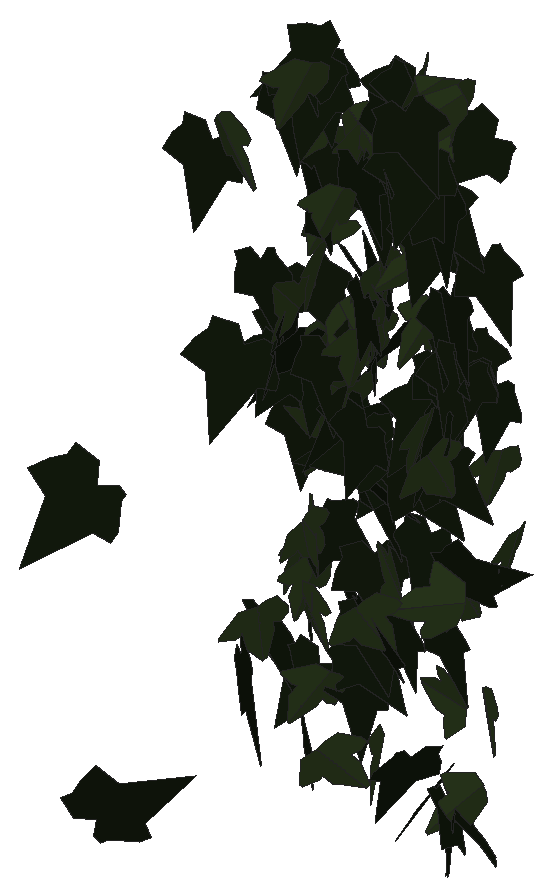
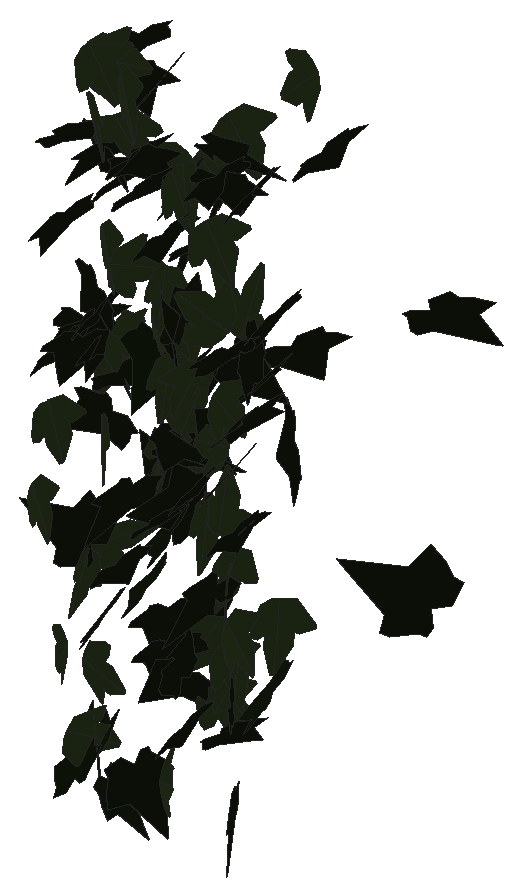
# SketchUp Ruby script. Lengths in inches.
U = 1.inch
M = Sketchup.active_model
def pt(a) = Geom::Point3d.new(a.map { |v| v * U })
def face(e, loops, mat)
  f = e.add_face(loops[0].map { |a| pt(a) })
  loops[1..].each { |l| e.add_face(l.map { |a| pt(a) }).erase! }
  f.material = f.back_material = mat if mat
  f
end
# faces: each face lists its corners as indices into pts; further lists are holes
def faces(e, pts, list, mat = nil) = list.each { |f| face(e, (f[0].is_a?(Array) ? f : [f]).map { |l| l.map { |i| pts[i] } }, mat) }
# xy, xz, yz: faces in a plane at the given z, y or x. An outline is a flat list of corners, or four numbers for a rectangle; further outlines are holes
def ring(l) = l.size == 4 ? [[l[0], l[1]], [l[2], l[1]], [l[2], l[3]], [l[0], l[3]]] : l.each_slice(2).to_a
def flat(e, list, mat, &to3) = list.each { |f| face(e, (f[0].is_a?(Array) ? f : [f]).map { |l| ring(l).map { |u, v| to3.(u, v) } }, mat) }
def xy(e, z, list, mat = nil) = flat(e, list, mat) { |x, y| [x, y, z] }
def xz(e, y, list, mat = nil) = flat(e, list, mat) { |x, z| [x, y, z] }
def yz(e, x, list, mat = nil) = flat(e, list, mat) { |y, z| [x, y, z] }
def lines(e, pts, list) = list.each { |a, b| e.add_line(pt(pts[a]), pt(pts[b])) }
# prism: a flat outline (further loops are holes) pulled along v
def prism(e, loops, v, mat = nil)
  f = face(e, loops, mat); d = Geom::Vector3d.new(v.map { |x| x * U })
  f.pushpull(f.normal.samedirection?(d) ? d.length : -d.length)
end
def box(e, o, s, mat = nil) = prism(e, [[o, [o[0] + s[0], o[1], o[2]], [o[0] + s[0], o[1] + s[1], o[2]], [o[0], o[1] + s[1], o[2]]]], [0, 0, s[2]], mat)
def at(x, y, z, deg = 0) = Geom::Transformation.translation(pt([x, y, z])) * Geom::Transformation.rotation(ORIGIN, Z_AXIS, deg.degrees)
def axes(o, x, y, z) = Geom::Transformation.new([*x, 0, *y, 0, *z, 0, *pt(o).to_a, 1])
def part(name) = M.definitions.add(name)
# library, detail: a bought-in or finely detailed component or shape, given as its bounding box
def library(name, o, s) = part(name).tap { |d| box(d.entities, o, s) }
def detail(e, o, s) = box(e.add_group.entities, o, s)
def put(e, d, t, mat = nil) = e.add_instance(d, t).tap { |i| i.material = mat if mat }
def group(e, t, mat = nil) = e.add_group.tap { |g| g.transformation = t; g.material = mat if mat }.entities
root = M.entities
M.materials.add("efeu1").color = [18, 25, 13]
M.materials.add("efeu2").color = [43, 57, 29]
c1 = part("ivyleaf_9")
p = [[1.54,2.16,1.25],[1.36,2.04,1.19],[-0.21,0.99,0.68],[-0.71,1.11,0.82],[-0.85,0.86,0.67],[-0.8,0.17,0.21],
  [-0.9,-0.01,0.1],[-0.67,-0.16,-0.02],[-0.08,-0.08,-0.05],[-0.03,-0.6,-0.4],[0.65,-0.88,-0.66],[0.83,-0.6,-0.49],
  [1.29,-0.42,-0.43],[1.8125,-0.07,-0.26],[1.21,0.44,0.15]]
faces(c1.entities,p,[[0,1,2,3,4,5,6,7,8,9,10,11,12,13,14]],"efeu1")
c2 = part("ivyleaf_10")
p = [[0,0.5,-0.03],[-0.0625,2.02,-0.43],[-0.19,2.01,-0.46],[-0.54,1.05,-0.29],[-0.52,0.625,-0.18],[-0.83,0.76,-0.28],
  [-1.16,0.64,-0.33],[-1.15,0.33,-0.24],[-0.77,-0.39,0.02],[-0.3,-0.51,0.16],[0.04,-0.48,0.23],[-0.02,2.01,-0.4375],
  [-0.06,2.01,-0.43],[0.04,-0.49,0.23],[0.67,-0.49,0.14],[1.38,0.36,-0.2],[1.375,0.51,-0.24],[0.81,0.65,-0.19],
  [0.62,0.59,-0.15],[0.6,1.09,-0.28],[0.5,1.23,-0.31]]
faces(c2.entities,p,[[0,1,2,3,4,5,6,7,8,9,10],[11,12,0,13,14,15,16,17,18,19,20]],"efeu2")
put(root,c1,axes([545.9,127.8,257.82],[-0.0474,-1.08135,0.06935],[0.00805,-0.06976,-1.08233],[1.08354,-0.04678,0.01108]))
put(root,c1,axes([545.62,125.77,249.51],[0.68735,-1.06043,0.13032],[0.07087,-0.10937,-1.26371],[1.06606,0.69099,-0.00001]))
put(root,c2,axes([546.39,127.24,252.71],[0.21842,-1.05759,0.41737],[0.07498,-0.41068,-1.07988],[1.1345,0.23076,-0.00898]))
put(root,c1,axes([546.03,127.84,249.28],[-0.01972,0.14168,1.08472],[0.16913,-1.07146,0.14302],[1.08078,0.17025,-0.00259]))
put(root,c1,axes([546.44,126.48,262.09],[-0.37568,-0.84617,0.61729],[-0.14119,-0.6089,-0.92059],[1.03784,-0.38913,0.09821]))
put(root,c1,axes([546.93,126.5,244.42],[0.34466,0.02289,-1.06433],[-1.01753,0.33599,-0.32228],[0.31299,1.0671,0.12431]))
put(root,c2,axes([546.76,127.19,251.46],[-0.20025,-0.98394,0.3749],[0.03102,-0.38696,-0.99904],[1.05248,-0.17581,0.10077]))
put(root,c1,axes([546.37,121.46,272.54],[-0.15743,-1.23369,0.2559],[-0.02108,-0.25528,-1.24364],[1.25977,-0.15844,0.01116]))
put(root,c1,axes([547.15,113.28,261.3125],[-1.10545,-0.855,0.27966],[-0.22516,-0.16598,-1.3975],[0.87094,-1.12813,-0.00633]))
put(root,c1,axes([546.27,127.41,260.47],[0.53298,-0.92924,-0.2297],[-0.03212,0.2454,-1.06727],[0.95667,0.52593,0.09214]))
put(root,c1,axes([546.39,126.1,272.68],[0.23212,-1.09957,0.10858],[0.01112,-0.10862,-1.12374],[1.10486,0.2321,-0.0115]))
put(root,c2,axes([546.68,126.86,250.51],[-0.9404,0.436,-0.41275],[0.36003,-0.20429,-1.03608],[-0.48045,-1.00647,0.0315]))
put(root,c2,axes([547.04,127.15,257.68],[-1.11811,0.08461,0.04764],[0.04353,-0.05549,1.1201],[0.0868,1.11775,0.05201]))
put(root,c1,axes([546.63,124.22,266.14],[0.32667,-1.06419,-0.17164],[-0.04146,0.16682,-1.11316],[1.07715,0.32916,0.00921]))
put(root,c1,axes([547.23,126.87,247.55],[-0.57367,-0.83343,0.32274],[-0.05716,-0.3485,-1.00157],[0.89191,-0.5584,0.14339]))
put(root,c2,axes([547.32,123.13,251.44],[-0.47793,-1.09363,-0.23784],[0.08557,0.22216,-1.19346],[1.11592,-0.48542,-0.01035]))
put(root,c1,axes([547.9375,126.61,274.55],[-1.07082,-0.1366,0.39034],[-0.37776,-0.11783,-1.07754],[0.1683,-1.13364,0.06496]))
put(root,c2,axes([547.64,127.13,270.79],[-0.50231,-0.92838,0.38137],[-0.19562,-0.32772,-1.05545],[0.98441,-0.53885,-0.01514]))
put(root,c1,axes([547.3,122.21,263.53],[-0.63807,-1.16576,0.00062],[0.00354,-0.00265,-1.32895],[1.16576,-0.63807,0.00437]))
put(root,c1,axes([547.15,127.42,273.74],[0.0073,-1.11482,-0.15801],[0.02033,0.15812,-1.11464],[1.12578,0.00437,0.02115]))
put(root,c1,axes([547.48,126.79,273.34],[-0.83367,-0.67955,-0.38777],[0.38547,0.13637,-1.06769],[0.68086,-0.90927,0.12968]))
put(root,c2,axes([547.68,126.52,260.64],[0.32349,-0.58164,0.93153],[-0.35772,0.86234,0.66266],[-1.03831,-0.4783,0.06192]))
put(root,c2,axes([547.42,127.07,266.66],[-0.12351,-0.9066,0.74321],[0.20806,0.7185,0.91105],[-1.15369,0.22663,0.08473]))
put(root,c2,axes([547.82,127.06,257.63],[-0.06391,-1.06831,-0.50269],[0.04264,0.50101,-1.07016],[1.1799,-0.07597,0.01145]))
put(root,c2,axes([547.82,126.26,262.43],[0.04476,-0.90283,0.65318],[0.12248,-0.64576,-0.90097],[1.10759,0.1079,0.07323]))
put(root,c2,axes([548.14,124.99,274.64],[-0.40515,-1.07486,0.48397],[-0.14799,-0.46133,-1.14847],[1.16947,-0.43075,0.02234]))
put(root,c1,axes([547.51,126.46,261.09],[0.03013,-1.0575,0.33625],[0.04169,-0.33506,-1.05749],[1.10889,0.04133,0.03062]))
put(root,c2,axes([548.34,125.27,253.58],[-0.31173,0.61857,-0.93908],[-0.40539,0.84714,0.69258],[1.04888,0.51126,-0.01141]))
put(root,c1,axes([547.7,124.18,262.3],[-0.21732,-0.89513,0.63774],[0.01797,-0.6529,-0.91027],[1.09893,-0.16634,0.141]))
put(root,c2,axes([547.99,125.15,254.59],[-0.19888,-0.90444,-0.56599],[0.20077,0.53373,-0.92343],[1.04788,-0.27392,0.06951]))
put(root,c1,axes([547.51,126.28,265.03],[0.25381,-0.99051,-0.46726],[0.15823,0.50778,-0.99045],[1.0837,0.15785,0.25405]))
put(root,c1,axes([547.84,126.62,254.05],[0.29675,-0.38248,-1.01683],[-0.30445,0.98256,-0.45844],[1.04285,0.39569,0.15551]))
put(root,c1,axes([547.92,124.38,264.2],[-0.43111,0.29112,-1.14791],[0.92868,-0.67493,-0.51995],[-0.73486,-1.02374,0.01635]))
put(root,c1,axes([548.54,124.3,263.38],[-0.4331,0.45574,-0.93139],[0.34463,-0.88872,-0.59511],[-0.97796,-0.51501,0.20276]))
put(root,c1,axes([547.94,127.95,259.16],[0.03261,-1.04881,0.30759],[0.04091,-0.30634,-1.04889],[1.09222,0.04278,0.0301]))
put(root,c2,axes([548.76,125.29,248.15],[-0.5097,-0.76914,0.62804],[-0.34704,-0.52344,-0.92269],[0.93036,-0.61663,-0.00011]))
put(root,c2,axes([548.44,124.1,265.05],[-0.11317,-0.84043,-0.93885],[-0.07432,-0.93654,0.84732],[-1.25787,0.13095,0.03441]))
put(root,c1,axes([547.77,112.95,247.21],[0.14459,-0.08116,1.41192],[1.4047,0.17295,-0.13391],[-0.16413,1.40873,0.09778]))
put(root,c1,axes([548.83,126.88,269.83],[-0.42252,-0.9618,0.39733],[0.02151,-0.43681,-1.03449],[1.04041,-0.38156,0.18275]))
put(root,c2,axes([548.51,119.78,274.61],[-0.78275,0.49504,-0.82855],[0.68865,-0.46098,-0.92602],[-0.67625,-1.04244,0.01603]))
put(root,c2,axes([548.96,126.5,263.64],[0.2266,1.03358,0.42909],[0.08967,0.41962,-1.05812],[-1.11551,0.24369,0.0021]))
put(root,c1,axes([548.96,127.28,247.41],[0.13371,-1.13293,0.15237],[-0.00544,-0.15404,-1.14056],[1.14312,0.13178,-0.02325]))
put(root,c2,axes([549.43,124.35,267.51],[0.41473,-1.03962,0.30394],[0.13784,-0.27215,-1.11898],[1.07433,0.43624,0.02624]))
put(root,c1,axes([549.46,124.78,262.9],[0.05441,-1.11069,-0.05596],[0.00028,0.05604,-1.11202],[1.1121,0.05433,0.00302]))
put(root,c2,axes([549.95,126.46,272.02],[-0.03503,-1.11742,0.22972],[-0.00028,-0.22982,-1.11795],[1.14079,-0.03436,0.00678]))
put(root,c1,axes([549.55,127.52,252.82],[-0.19804,-1.00307,-0.49728],[0.13617,0.47967,-1.02178],[1.11126,-0.23754,0.03658]))
put(root,c1,axes([549.1,127.33,249.89],[0.2571,-0.38242,1.05071],[0.59166,-0.8683,-0.4608],[0.94878,0.6451,0.00263]))
put(root,c1,axes([550.27,125.74,260.3],[0.042,0.35924,-1.0748],[-0.05967,-1.07335,-0.36108],[-1.13168,0.06993,-0.02085]))
put(root,c2,axes([550.05,125.86,260.7],[-0.22719,-0.68738,-0.8885],[-0.15821,-0.87788,0.71962],[-1.11216,0.2653,0.07913]))
put(root,c1,axes([550.01,128.11,256.92],[-0.44564,-0.85693,0.48361],[-0.00704,-0.5281,-0.94227],[0.98395,-0.39189,0.21228]))
put(root,c2,axes([550.15,126.68,263.46],[-0.22297,-1.02658,-0.33738],[0.14562,0.3128,-1.04803],[1.07074,-0.25631,0.07228]))
put(root,c1,axes([549.91,126.94,250.8],[-0.16228,-0.99267,-0.47818],[0.13225,0.46229,-1.00458],[1.09387,-0.20316,0.05052]))
put(root,c1,axes([549.64,126.52,249.36],[-0.10965,-0.53448,-0.92771],[0.64659,0.71024,-0.48561],[0.85337,-0.60682,0.24874]))
put(root,c2,axes([549.81,127.41,244.59],[0.26555,-0.51544,0.98689],[0.69955,-0.71205,-0.56012],[0.86617,0.7331,0.14983]))
put(root,c1,axes([549.42,126.17,257.12],[0.95005,-0.32352,0.53916],[0.50631,-0.18567,-1.00356],[0.37285,1.07648,-0.01106]))
put(root,c1,axes([549.53,126.52,265.8],[0.28041,-0.58159,0.91123],[0.57877,-0.71432,-0.63402],[0.91302,0.63144,0.12205]))
put(root,c1,axes([551.16,125.64,258.96],[-0.90507,-0.05997,0.71402],[-0.71223,-0.05071,-0.90705],[0.07849,-1.1517,0.00275]))
put(root,c1,axes([549.9,123.81,269.97],[-0.02899,-0.47694,1.18997],[0.09116,-1.18803,-0.47394],[1.27875,0.07388,0.06076]))
put(root,c1,axes([549.76,127.14,256.125],[0.58137,-0.89238,0.22109],[0.10012,-0.19858,-1.06478],[0.9139,0.58944,-0.024]))
put(root,c1,axes([551.07,126.08,264.9],[0.01359,-0.08953,1.1406],[-0.43069,1.05637,0.08805],[-1.05994,-0.43039,-0.02116]))
put(root,c2,axes([549.97,126.07,272.75],[-0.79452,0.06631,-0.84981],[0.78572,-0.39343,-0.7653],[-0.33047,-1.09483,0.22355]))
put(root,c1,axes([550.27,126.96,269.75],[0.02217,-1.12343,-0.05151],[0.00323,0.05158,-1.12364],[1.12461,0.022,0.00424]))
put(root,c1,axes([550.93,128.11,273.6],[-0.81682,-0.76542,0.12972],[-0.10397,-0.07874,-1.11932],[0.76934,-0.8233,-0.01355]))
put(root,c1,axes([550.26,126.39,264.58],[-0.37043,0.05683,-1.14627],[1.13111,-0.1858,-0.37475],[-0.19426,-1.19022,0.00377]))
put(root,c1,axes([550.66,128.32,272.25],[-0.35257,-0.96913,0.4354],[0.00384,-0.45991,-1.02057],[1.06244,-0.31994,0.14818]))
put(root,c2,axes([551.18,123.07,271.02],[-0.23652,-0.95803,0.59751],[0.00244,-0.61091,-0.97855],[1.12908,-0.19937,0.12728]))
put(root,c2,axes([551.12,125.78,266.8],[-0.12658,-1.03452,-0.43706],[0.07337,0.43127,-1.04207],[1.12066,-0.14509,0.01886]))
put(root,c1,axes([550.55,125.28,271.23],[0.48781,-1.02484,0.12803],[0.0368,-0.12425,-1.13483],[1.03215,0.48878,-0.02005]))
put(root,c1,axes([551.42,127.3125,244.68],[-0.0952,0.85584,-0.73902],[0.10415,-0.73185,-0.86094],[-1.12595,-0.14005,-0.01715]))
put(root,c2,axes([551.32,124.46,264.4],[-0.3668,-1.04887,0.15004],[-0.03142,-0.14794,-1.11099],[1.05908,-0.36766,0.019]))
put(root,c1,axes([551.43,125.96,263.45],[0.12728,0.99317,0.60816],[0.05552,0.60591,-1.00112],[-1.16326,0.13759,0.01876]))
put(root,c1,axes([551.02,128.1875,273.57],[-0.32658,-1.01037,0.36855],[0.00379,-0.38624,-1.05553],[1.07549,-0.30545,0.11563]))
put(root,c2,axes([551.12,126.21,265.16],[0.50139,-0.90225,0.51215],[0.29509,-0.4213,-1.0311],[0.99462,0.57982,0.04774]))
put(root,c1,axes([551.83,128.01,254.32],[-0.16942,-1.05432,0.10786],[-0.0177,-0.1064,-1.06784],[1.05967,-0.17034,-0.00059]))
put(root,c1,axes([552.47,127.625,243.78],[-0.62243,0.63623,-0.49306],[0.25209,-0.43784,-0.88321],[-0.76443,-0.66243,0.11021]))
put(root,c1,axes([551.73,127.22,257.6],[0.28387,-0.80489,-0.85135],[-0.10511,0.85495,-0.84334],[1.16687,0.27282,0.13114]))
put(root,c1,axes([551.57,124.3125,266.16],[0.44224,-0.21275,-1.09936],[0.95912,-0.53804,0.48994],[-0.57789,-1.05579,-0.02816]))
put(root,c1,axes([552.0625,123.84,260.9],[-0.07612,-1.00887,0.49826],[-0.04549,-0.49624,-1.01171],[1.12429,-0.08838,-0.0072]))
put(root,c2,axes([552.28,127.3125,264.4],[-0.17764,-0.61445,0.90299],[0.26562,-0.91169,-0.56812],[1.05943,0.12555,0.29385]))
put(root,c2,axes([552.59,126.7,267.36],[-0.13146,-0.30689,1.0629],[-0.13912,-1.05729,-0.32247],[1.09753,-0.17078,0.08643]))
put(root,c2,axes([552.65,126.4375,275.52],[0.40685,-1.06826,-0.1193],[-0.03628,0.11384,-1.14309],[1.07428,0.40842,0.00657]))
put(root,c2,axes([552.43,120.97,248.05],[-0.66283,-0.64825,-0.76951],[0.53846,0.54989,-0.92705],[0.84996,-0.85389,-0.01281]))
put(root,c1,axes([552.375,125.46,251.91],[0.3641,-0.95835,0.35796],[0.15719,-0.32303,-1.02473],[1.01087,0.39541,0.03042]))
put(root,c2,axes([553.14,127.04,268.61],[0.43102,-1.02813,-0.17206],[-0.03286,0.17269,-1.11424],[1.04191,0.43077,0.03603]))
put(root,c2,axes([553.32,125.79,273.32],[1.09996,0.29562,-0.47888],[-0.45999,-0.13347,-1.13896],[-0.32424,1.19224,-0.00877]))
put(root,c1,axes([552.45,115.76,254.4375],[-0.18204,0.02579,-1.46881],[1.45789,-0.1788,-0.18382],[-0.18062,-1.46921,-0.00341]))
put(root,c2,axes([554.05,126.77,248.34],[0.10539,-0.0531,-1.15192],[-0.98139,0.60323,-0.11759],[0.60548,0.98698,0.0099]))
put(root,c1,axes([552.88,124.41,274.47],[0.14942,-1.09403,0.44387],[0.09832,-0.43433,-1.1036],[1.17654,0.17523,0.03585]))
put(root,c2,axes([553.73,123.4,254.82],[-0.63673,0.92811,0.25923],[0.13844,-0.21938,1.12549],[0.95364,0.65153,0.0097]))
put(root,c1,axes([553.71,125.75,261.63],[-0.61724,-0.89334,0.26512],[-0.07253,-0.27098,-1.08196],[0.92902,-0.61469,0.09168]))
put(root,c1,axes([553.15,127.18,251.13],[0.49791,-0.97704,0.03663],[-0.00219,-0.04222,-1.09639],[0.97773,0.49746,-0.02111]))
put(root,c2,axes([553.95,126.95,274.47],[0.62668,-0.76033,-0.53499],[-0.3122,0.4356,-0.98479],[0.8757,0.69942,0.03176]))
put(root,c2,axes([553.83,126.33,259.2],[0.60284,-0.73352,-0.57743],[-0.14245,0.60703,-0.91985],[0.9226,0.57302,0.23528]))
put(root,c1,axes([553.64,127.11,265.03],[0.03395,-1.06748,0.33836],[0.00177,-0.33846,-1.06798],[1.11982,0.0329,-0.00857]))
put(root,c2,axes([554.11,127.09,253.17],[0.15862,-0.89196,-0.66582],[0.14139,0.68325,-0.88162],[1.10405,0.04064,0.20856]))
put(root,c2,axes([554.55,125.71,253.33],[-0.06359,0.24107,1.20612],[-0.32083,-1.16917,0.21677],[1.1874,-0.30299,0.12317]))
put(root,c1,axes([553.86,126.13,263.38],[0.25844,-1.0281,-0.34019],[-0.1068,0.32384,-1.05983],[1.07765,0.27865,-0.02345]))
put(root,c1,axes([553.91,126.73,265.92],[-0.37516,-0.16215,-1.07741],[1.07593,0.12445,-0.39338],[0.17172,-1.13405,0.11089]))
put(root,c2,axes([554.87,125.32,275.58],[-0.2697,-0.39232,1.1537],[-0.25144,-1.13827,-0.44586],[1.19236,-0.32877,0.16694]))
put(root,c1,axes([554.16,127.34,263.74],[-0.18972,-0.94602,-0.63753],[0.22084,0.60361,-0.9614],[1.11921,-0.27946,0.08163]))
put(root,c2,axes([554.84,125.68,275.94],[-0.2895,-1.06706,0.39731],[-0.12744,-0.37701,-1.1054],[1.13147,-0.31548,-0.02285]))
put(root,c1,axes([554.38,125.92,242.32],[-0.15732,0.45568,0.90404],[0.08528,-0.90567,0.47135],[1.00879,0.14762,0.10114]))
put(root,c2,axes([554.93,126.64,244.7],[-0.22596,-0.41598,0.99444],[-0.07793,-1.00709,-0.43898],[1.07511,-0.16043,0.17719]))
put(root,c1,axes([554.44,124.76,269.96],[-0.15439,-1.07995,0.41912],[0.04534,-0.42813,-1.08648],[1.15754,-0.12727,0.09846]))
put(root,c1,axes([554.46,126.01,243.87],[-0.01944,-0.57224,0.85225],[0.16724,-0.84278,-0.56207],[1.01283,0.12817,0.10917]))
put(root,c1,axes([555.13,127.66,273.06],[-0.7803,-0.67046,0.46791],[-0.17738,-0.49258,-1.00161],[0.79812,-0.76496,0.23486]))
put(root,c2,axes([554.94,123.75,262.19],[0.29463,-1.08245,0.19778],[0.06531,-0.18718,-1.12175],[1.09843,0.30147,0.01365]))
put(root,c2,axes([554.83,120.15,255.4],[-0.66045,-0.83169,-0.62451],[0.37947,0.4961,-1.06198],[0.96836,-0.76164,-0.00977]))
put(root,c1,axes([554.21,125.5,259.51],[0.03803,-0.3789,-1.04799],[0.84772,0.69048,-0.21887],[0.72334,-0.78928,0.31161]))
put(root,c1,axes([555.07,124.62,261.99],[-0.93304,0.17916,-0.7124],[0.70547,-0.10242,-0.94973],[-0.20473,-1.16943,-0.02596]))
put(root,c1,axes([554.58,123.2,275.89],[0.1075,-1.03952,-0.5103],[0.12231,0.51982,-1.03315],[1.15154,0.04183,0.15737]))
put(root,c1,axes([555.14,123.34,274.09],[-0.83572,-0.86228,-0.29175],[0.19394,0.21831,-1.20076],[0.8894,-0.85784,-0.01231]))
put(root,c1,axes([554.8125,126.99,243.05],[0.90543,-0.64183,-0.32418],[0.26285,-0.18977,1.10984],[-0.66929,-0.94281,-0.0027]))
put(root,c1,axes([555.08,126.18,263.69],[-0.34668,-1.12972,0.06879],[-0.01415,-0.06761,-1.1817],[1.13173,-0.34691,0.00629]))
put(root,c1,axes([554.6875,124.79,271.55],[0.33334,-0.92086,-0.61342],[0.12819,0.66848,-0.93386],[1.09902,0.20133,0.29498]))
put(root,c1,axes([554.32,126.77,253.9375],[0.28498,-0.16166,1.12772],[1.07203,-0.35534,-0.32184],[0.38554,1.10757,0.06135]))
put(root,c1,axes([555.21,125.875,263.67],[-0.80406,-0.63244,-0.46672],[0.35733,0.30056,-1.02289],[0.70009,-0.87978,-0.01395]))
put(root,c1,axes([554.89,125.0625,271.45],[-0.54775,-0.26962,-1.00386],[1.02811,0.02656,-0.56811],[0.15306,-1.14327,0.22354]))
put(root,c1,axes([554.51,121.39,253.84],[0.21206,-0.54738,1.23379],[0.65447,-1.05059,-0.57859],[1.18048,0.68079,0.09914]))
put(root,c2,axes([555.46,127.02,248.81],[-0.6185,0.58485,-0.59444],[0.29374,-0.53987,-0.83678],[-0.78047,-0.66667,0.15614]))
put(root,c2,axes([555.92,127.15,259.54],[-0.30778,-1.0108,0.14745],[-0.03326,-0.144,-1.05657],[1.02096,-0.30941,0.01003]))
put(root,c2,axes([555.85,123.07,261.17],[-0.34506,-1.0191,-0.60265],[0.22208,0.56087,-1.0756],[1.16294,-0.40948,0.02659]))
put(root,c1,axes([555.77,127.13,262.61],[-0.00956,-1.06825,0.28735],[-0.02267,-0.28711,-1.06812],[1.10599,-0.01512,-0.01941]))
put(root,c2,axes([556.21,127.72,255.87],[0.22811,-1.02347,0.10611],[0.02756,-0.10257,-1.04857],[1.02858,0.22972,0.00457]))
put(root,c1,axes([555.88,126.39,268.49],[0.20861,-1.05238,-0.35762],[-0.00696,0.36262,-1.07116],[1.11146,0.19979,0.06042]))
